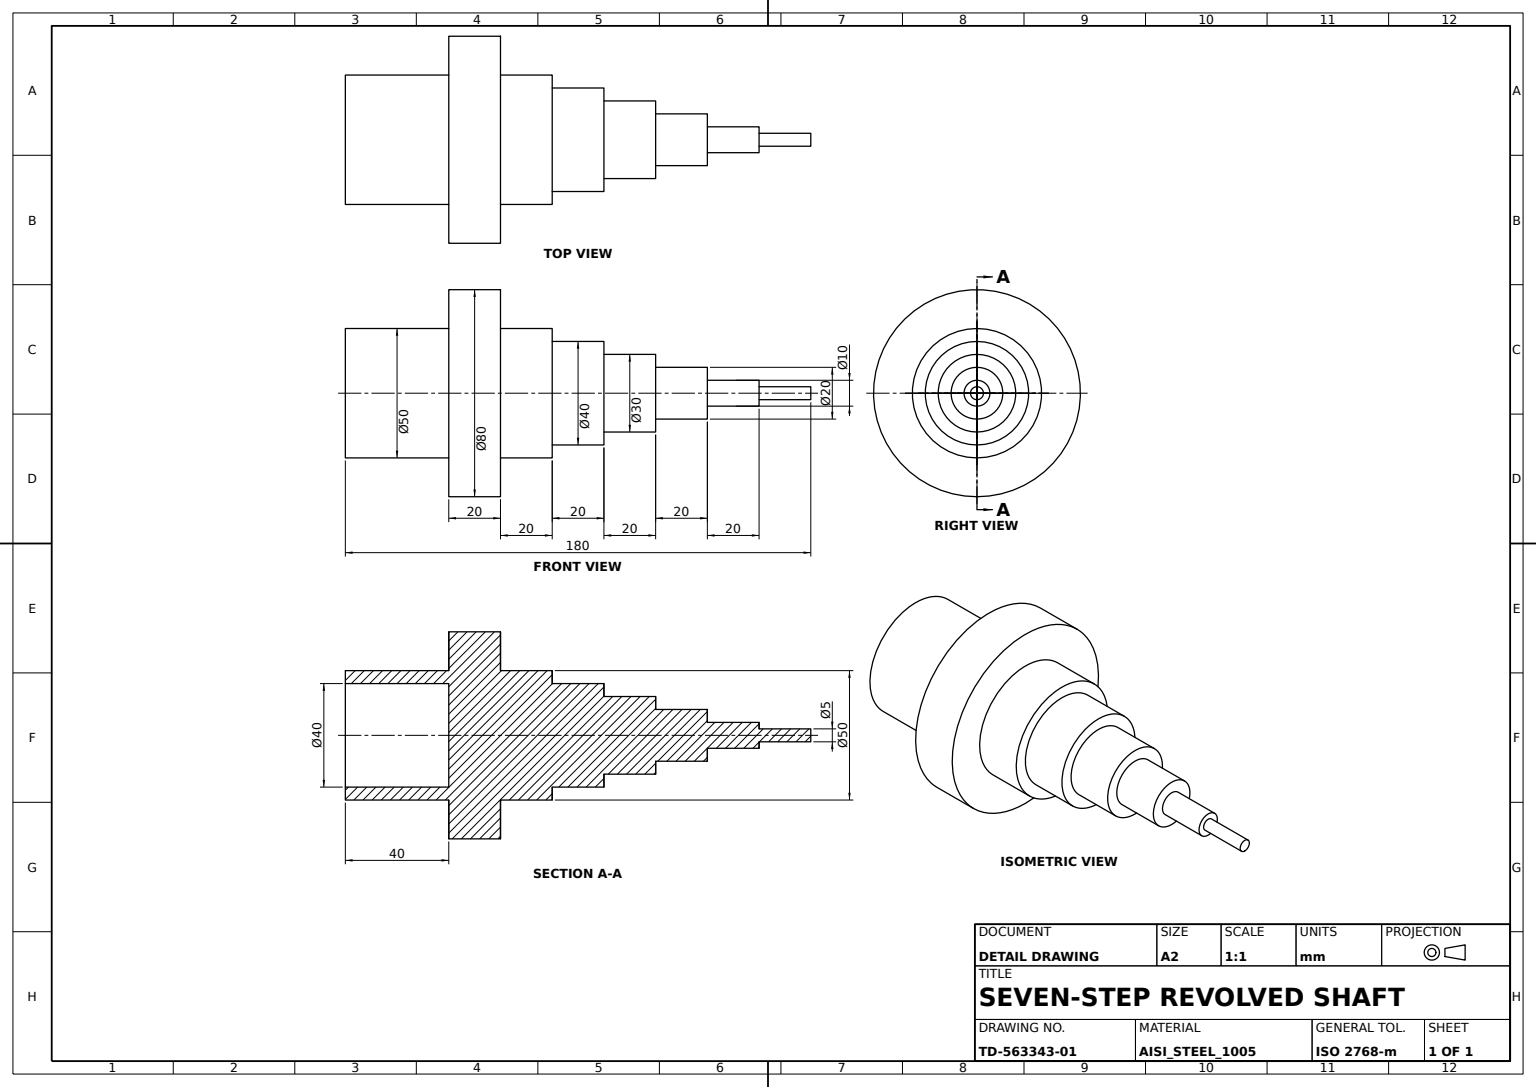
ISO-10303-21;
HEADER;
FILE_DESCRIPTION((''),'2;1');
FILE_NAME('','',(''),(''),'','','');
FILE_SCHEMA(('AUTOMOTIVE_DESIGN'));
ENDSEC;
DATA;
#1=APPLICATION_CONTEXT('');
#2=PRODUCT_CONTEXT('',#1,'mechanical');
#3=PRODUCT('','','',(#2));
#4=PRODUCT_DEFINITION_FORMATION('','',#3);
#5=PRODUCT_DEFINITION_CONTEXT('',#1,'design');
#6=PRODUCT_DEFINITION('','',#4,#5);
#7=PRODUCT_DEFINITION_SHAPE('','',#6);
#8=(LENGTH_UNIT()NAMED_UNIT(*)SI_UNIT(.MILLI.,.METRE.));
#9=(NAMED_UNIT(*)PLANE_ANGLE_UNIT()SI_UNIT($,.RADIAN.));
#10=(NAMED_UNIT(*)SI_UNIT($,.STERADIAN.)SOLID_ANGLE_UNIT());
#11=UNCERTAINTY_MEASURE_WITH_UNIT(LENGTH_MEASURE(0.005),#8,'distance_accuracy_value','');
#12=(GEOMETRIC_REPRESENTATION_CONTEXT(3)GLOBAL_UNCERTAINTY_ASSIGNED_CONTEXT((#11))GLOBAL_UNIT_ASSIGNED_CONTEXT((#8,#9,#10))REPRESENTATION_CONTEXT('',''));
#13=CARTESIAN_POINT('',(140.,0.,-10.));
#14=VERTEX_POINT('',#13);
#15=CARTESIAN_POINT('',(140.,0.,0.));
#16=DIRECTION('',(1.,0.,0.));
#17=DIRECTION('',(0.,0.,-1.));
#18=AXIS2_PLACEMENT_3D('',#15,#16,#17);
#19=CIRCLE('',#18,10.);
#20=EDGE_CURVE('',#14,#14,#19,.T.);
#21=ORIENTED_EDGE('',*,*,#20,.F.);
#22=EDGE_LOOP('',(#21));
#23=FACE_BOUND('',#22,.T.);
#24=CARTESIAN_POINT('',(120.,0.,-10.));
#25=VERTEX_POINT('',#24);
#26=CARTESIAN_POINT('',(120.,0.,0.));
#27=AXIS2_PLACEMENT_3D('',#26,#16,#17);
#28=CIRCLE('',#27,10.);
#29=EDGE_CURVE('',#25,#25,#28,.T.);
#30=ORIENTED_EDGE('',*,*,#29,.T.);
#31=EDGE_LOOP('',(#30));
#32=FACE_BOUND('',#31,.T.);
#33=CARTESIAN_POINT('',(0.,0.,0.));
#34=AXIS2_PLACEMENT_3D('',#33,#16,#17);
#35=CYLINDRICAL_SURFACE('',#34,10.);
#36=ADVANCED_FACE('',(#23,#32),#35,.T.);
#37=CARTESIAN_POINT('',(160.,0.,-2.5));
#38=VERTEX_POINT('',#37);
#39=CARTESIAN_POINT('',(160.,0.,0.));
#40=AXIS2_PLACEMENT_3D('',#39,#16,#17);
#41=CIRCLE('',#40,2.5);
#42=EDGE_CURVE('',#38,#38,#41,.T.);
#43=ORIENTED_EDGE('',*,*,#42,.T.);
#44=EDGE_LOOP('',(#43));
#45=FACE_BOUND('',#44,.T.);
#46=CARTESIAN_POINT('',(180.,0.,-2.5));
#47=VERTEX_POINT('',#46);
#48=CARTESIAN_POINT('',(180.,0.,0.));
#49=AXIS2_PLACEMENT_3D('',#48,#16,#17);
#50=CIRCLE('',#49,2.5);
#51=EDGE_CURVE('',#47,#47,#50,.T.);
#52=ORIENTED_EDGE('',*,*,#51,.F.);
#53=EDGE_LOOP('',(#52));
#54=FACE_BOUND('',#53,.T.);
#55=CYLINDRICAL_SURFACE('',#34,2.5);
#56=ADVANCED_FACE('',(#45,#54),#55,.T.);
#57=ORIENTED_EDGE('',*,*,#20,.T.);
#58=EDGE_LOOP('',(#57));
#59=FACE_BOUND('',#58,.T.);
#60=CARTESIAN_POINT('',(140.,0.,-5.));
#61=VERTEX_POINT('',#60);
#62=CIRCLE('',#18,5.);
#63=EDGE_CURVE('',#61,#61,#62,.T.);
#64=ORIENTED_EDGE('',*,*,#63,.F.);
#65=EDGE_LOOP('',(#64));
#66=FACE_BOUND('',#65,.T.);
#67=CARTESIAN_POINT('',(140.,0.,5.));
#68=AXIS2_PLACEMENT_3D('',#67,#16,#17);
#69=PLANE('',#68);
#70=ADVANCED_FACE('',(#59,#66),#69,.T.);
#71=CARTESIAN_POINT('',(100.,0.,-15.));
#72=VERTEX_POINT('',#71);
#73=CARTESIAN_POINT('',(100.,0.,0.));
#74=AXIS2_PLACEMENT_3D('',#73,#16,#17);
#75=CIRCLE('',#74,15.);
#76=EDGE_CURVE('',#72,#72,#75,.T.);
#77=ORIENTED_EDGE('',*,*,#76,.F.);
#78=EDGE_LOOP('',(#77));
#79=FACE_BOUND('',#78,.T.);
#80=CARTESIAN_POINT('',(100.,0.,-20.));
#81=VERTEX_POINT('',#80);
#82=CIRCLE('',#74,20.);
#83=EDGE_CURVE('',#81,#81,#82,.T.);
#84=ORIENTED_EDGE('',*,*,#83,.T.);
#85=EDGE_LOOP('',(#84));
#86=FACE_BOUND('',#85,.T.);
#87=CARTESIAN_POINT('',(100.,0.,15.));
#88=AXIS2_PLACEMENT_3D('',#87,#16,#17);
#89=PLANE('',#88);
#90=ADVANCED_FACE('',(#79,#86),#89,.T.);
#91=CARTESIAN_POINT('',(40.,20.,0.));
#92=VERTEX_POINT('',#91);
#93=CARTESIAN_POINT('',(40.,0.,0.));
#94=DIRECTION('',(-1.,0.,0.));
#95=DIRECTION('',(0.,1.,0.));
#96=AXIS2_PLACEMENT_3D('',#93,#94,#95);
#97=CIRCLE('',#96,20.);
#98=EDGE_CURVE('',#92,#92,#97,.F.);
#99=ORIENTED_EDGE('',*,*,#98,.T.);
#100=EDGE_LOOP('',(#99));
#101=FACE_BOUND('',#100,.T.);
#102=CARTESIAN_POINT('',(0.,20.,0.));
#103=VERTEX_POINT('',#102);
#104=AXIS2_PLACEMENT_3D('',#33,#94,#95);
#105=CIRCLE('',#104,20.);
#106=EDGE_CURVE('',#103,#103,#105,.T.);
#107=ORIENTED_EDGE('',*,*,#106,.T.);
#108=EDGE_LOOP('',(#107));
#109=FACE_BOUND('',#108,.T.);
#110=DIRECTION('',(0.,0.,1.));
#111=AXIS2_PLACEMENT_3D('',#93,#94,#110);
#112=CYLINDRICAL_SURFACE('',#111,20.);
#113=ADVANCED_FACE('',(#101,#109),#112,.F.);
#114=ORIENTED_EDGE('',*,*,#76,.T.);
#115=EDGE_LOOP('',(#114));
#116=FACE_BOUND('',#115,.T.);
#117=CARTESIAN_POINT('',(120.,0.,-15.));
#118=VERTEX_POINT('',#117);
#119=CIRCLE('',#27,15.);
#120=EDGE_CURVE('',#118,#118,#119,.T.);
#121=ORIENTED_EDGE('',*,*,#120,.F.);
#122=EDGE_LOOP('',(#121));
#123=FACE_BOUND('',#122,.T.);
#124=CYLINDRICAL_SURFACE('',#34,15.);
#125=ADVANCED_FACE('',(#116,#123),#124,.T.);
#126=CARTESIAN_POINT('',(80.,0.,-20.));
#127=VERTEX_POINT('',#126);
#128=CARTESIAN_POINT('',(80.,0.,0.));
#129=AXIS2_PLACEMENT_3D('',#128,#16,#17);
#130=CIRCLE('',#129,20.);
#131=EDGE_CURVE('',#127,#127,#130,.T.);
#132=ORIENTED_EDGE('',*,*,#131,.F.);
#133=EDGE_LOOP('',(#132));
#134=FACE_BOUND('',#133,.T.);
#135=CARTESIAN_POINT('',(80.,0.,-25.));
#136=VERTEX_POINT('',#135);
#137=CIRCLE('',#129,25.);
#138=EDGE_CURVE('',#136,#136,#137,.T.);
#139=ORIENTED_EDGE('',*,*,#138,.T.);
#140=EDGE_LOOP('',(#139));
#141=FACE_BOUND('',#140,.T.);
#142=CARTESIAN_POINT('',(80.,0.,20.));
#143=AXIS2_PLACEMENT_3D('',#142,#16,#17);
#144=PLANE('',#143);
#145=ADVANCED_FACE('',(#134,#141),#144,.T.);
#146=ORIENTED_EDGE('',*,*,#98,.F.);
#147=EDGE_LOOP('',(#146));
#148=FACE_BOUND('',#147,.T.);
#149=PLANE('',#111);
#150=ADVANCED_FACE('',(#148),#149,.T.);
#151=ORIENTED_EDGE('',*,*,#51,.T.);
#152=EDGE_LOOP('',(#151));
#153=FACE_BOUND('',#152,.T.);
#154=PLANE('',#49);
#155=ADVANCED_FACE('',(#153),#154,.T.);
#156=CARTESIAN_POINT('',(40.,0.,-25.));
#157=VERTEX_POINT('',#156);
#158=AXIS2_PLACEMENT_3D('',#93,#16,#17);
#159=CIRCLE('',#158,25.);
#160=EDGE_CURVE('',#157,#157,#159,.T.);
#161=ORIENTED_EDGE('',*,*,#160,.T.);
#162=EDGE_LOOP('',(#161));
#163=FACE_BOUND('',#162,.T.);
#164=CARTESIAN_POINT('',(40.,0.,-40.));
#165=VERTEX_POINT('',#164);
#166=CIRCLE('',#158,40.);
#167=EDGE_CURVE('',#165,#165,#166,.T.);
#168=ORIENTED_EDGE('',*,*,#167,.F.);
#169=EDGE_LOOP('',(#168));
#170=FACE_BOUND('',#169,.T.);
#171=CARTESIAN_POINT('',(40.,0.,40.));
#172=AXIS2_PLACEMENT_3D('',#171,#94,#110);
#173=PLANE('',#172);
#174=ADVANCED_FACE('',(#163,#170),#173,.T.);
#175=ORIENTED_EDGE('',*,*,#83,.F.);
#176=EDGE_LOOP('',(#175));
#177=FACE_BOUND('',#176,.T.);
#178=ORIENTED_EDGE('',*,*,#131,.T.);
#179=EDGE_LOOP('',(#178));
#180=FACE_BOUND('',#179,.T.);
#181=CYLINDRICAL_SURFACE('',#34,20.);
#182=ADVANCED_FACE('',(#177,#180),#181,.T.);
#183=CARTESIAN_POINT('',(60.,0.,-40.));
#184=VERTEX_POINT('',#183);
#185=CARTESIAN_POINT('',(60.,0.,0.));
#186=AXIS2_PLACEMENT_3D('',#185,#16,#17);
#187=CIRCLE('',#186,40.);
#188=EDGE_CURVE('',#184,#184,#187,.T.);
#189=ORIENTED_EDGE('',*,*,#188,.F.);
#190=EDGE_LOOP('',(#189));
#191=FACE_BOUND('',#190,.T.);
#192=ORIENTED_EDGE('',*,*,#167,.T.);
#193=EDGE_LOOP('',(#192));
#194=FACE_BOUND('',#193,.T.);
#195=CYLINDRICAL_SURFACE('',#34,40.);
#196=ADVANCED_FACE('',(#191,#194),#195,.T.);
#197=CARTESIAN_POINT('',(160.,0.,-5.));
#198=VERTEX_POINT('',#197);
#199=CIRCLE('',#40,5.);
#200=EDGE_CURVE('',#198,#198,#199,.T.);
#201=ORIENTED_EDGE('',*,*,#200,.F.);
#202=EDGE_LOOP('',(#201));
#203=FACE_BOUND('',#202,.T.);
#204=ORIENTED_EDGE('',*,*,#63,.T.);
#205=EDGE_LOOP('',(#204));
#206=FACE_BOUND('',#205,.T.);
#207=CYLINDRICAL_SURFACE('',#34,5.);
#208=ADVANCED_FACE('',(#203,#206),#207,.T.);
#209=ORIENTED_EDGE('',*,*,#188,.T.);
#210=EDGE_LOOP('',(#209));
#211=FACE_BOUND('',#210,.T.);
#212=CARTESIAN_POINT('',(60.,0.,-25.));
#213=VERTEX_POINT('',#212);
#214=CIRCLE('',#186,25.);
#215=EDGE_CURVE('',#213,#213,#214,.T.);
#216=ORIENTED_EDGE('',*,*,#215,.F.);
#217=EDGE_LOOP('',(#216));
#218=FACE_BOUND('',#217,.T.);
#219=CARTESIAN_POINT('',(60.,0.,25.));
#220=AXIS2_PLACEMENT_3D('',#219,#16,#17);
#221=PLANE('',#220);
#222=ADVANCED_FACE('',(#211,#218),#221,.T.);
#223=CARTESIAN_POINT('',(0.,0.,-25.));
#224=VERTEX_POINT('',#223);
#225=CIRCLE('',#34,25.);
#226=EDGE_CURVE('',#224,#224,#225,.T.);
#227=ORIENTED_EDGE('',*,*,#226,.T.);
#228=EDGE_LOOP('',(#227));
#229=FACE_BOUND('',#228,.T.);
#230=ORIENTED_EDGE('',*,*,#160,.F.);
#231=EDGE_LOOP('',(#230));
#232=FACE_BOUND('',#231,.T.);
#233=CYLINDRICAL_SURFACE('',#34,25.);
#234=ADVANCED_FACE('',(#229,#232),#233,.T.);
#235=ORIENTED_EDGE('',*,*,#106,.F.);
#236=EDGE_LOOP('',(#235));
#237=FACE_BOUND('',#236,.T.);
#238=ORIENTED_EDGE('',*,*,#226,.F.);
#239=EDGE_LOOP('',(#238));
#240=FACE_BOUND('',#239,.T.);
#241=CARTESIAN_POINT('',(0.,0.,25.));
#242=AXIS2_PLACEMENT_3D('',#241,#94,#110);
#243=PLANE('',#242);
#244=ADVANCED_FACE('',(#237,#240),#243,.T.);
#245=ORIENTED_EDGE('',*,*,#200,.T.);
#246=EDGE_LOOP('',(#245));
#247=FACE_BOUND('',#246,.T.);
#248=ORIENTED_EDGE('',*,*,#42,.F.);
#249=EDGE_LOOP('',(#248));
#250=FACE_BOUND('',#249,.T.);
#251=CARTESIAN_POINT('',(160.,0.,2.5));
#252=AXIS2_PLACEMENT_3D('',#251,#16,#17);
#253=PLANE('',#252);
#254=ADVANCED_FACE('',(#247,#250),#253,.T.);
#255=ORIENTED_EDGE('',*,*,#215,.T.);
#256=EDGE_LOOP('',(#255));
#257=FACE_BOUND('',#256,.T.);
#258=ORIENTED_EDGE('',*,*,#138,.F.);
#259=EDGE_LOOP('',(#258));
#260=FACE_BOUND('',#259,.T.);
#261=ADVANCED_FACE('',(#257,#260),#233,.T.);
#262=ORIENTED_EDGE('',*,*,#29,.F.);
#263=EDGE_LOOP('',(#262));
#264=FACE_BOUND('',#263,.T.);
#265=ORIENTED_EDGE('',*,*,#120,.T.);
#266=EDGE_LOOP('',(#265));
#267=FACE_BOUND('',#266,.T.);
#268=CARTESIAN_POINT('',(120.,0.,10.));
#269=AXIS2_PLACEMENT_3D('',#268,#16,#17);
#270=PLANE('',#269);
#271=ADVANCED_FACE('',(#264,#267),#270,.T.);
#272=CLOSED_SHELL('',(#36,#56,#70,#90,#113,#125,#145,#150,#155,#174,#182,#196,#208,#222,#234,#244,#254,#261,#271));
#273=MANIFOLD_SOLID_BREP('',#272);
#274=ADVANCED_BREP_SHAPE_REPRESENTATION('',(#273),#12);
#275=SHAPE_DEFINITION_REPRESENTATION(#7,#274);
ENDSEC;
END-ISO-10303-21;
